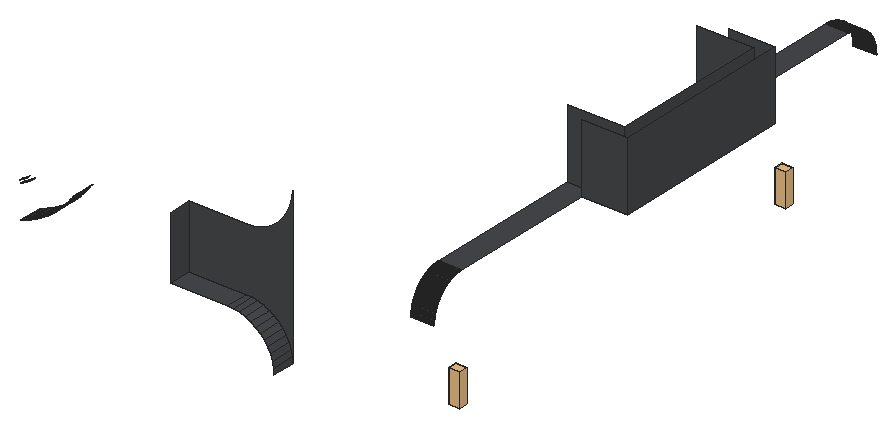
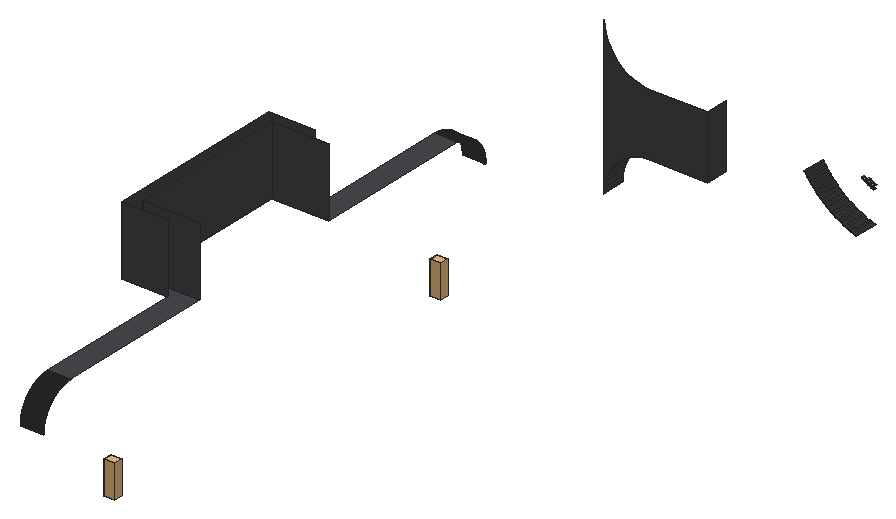
# SketchUp Ruby script. Lengths in inches.
U = 1.inch
M = Sketchup.active_model
def pt(a) = Geom::Point3d.new(a.map { |v| v * U })
def face(e, loops, mat)
  f = e.add_face(loops[0].map { |a| pt(a) })
  loops[1..].each { |l| e.add_face(l.map { |a| pt(a) }).erase! }
  f.material = f.back_material = mat if mat
  f
end
# faces: each face lists its corners as indices into pts; further lists are holes
def faces(e, pts, list, mat = nil) = list.each { |f| face(e, (f[0].is_a?(Array) ? f : [f]).map { |l| l.map { |i| pts[i] } }, mat) }
# xy, xz, yz: faces in a plane at the given z, y or x. An outline is a flat list of corners, or four numbers for a rectangle; further outlines are holes
def ring(l) = l.size == 4 ? [[l[0], l[1]], [l[2], l[1]], [l[2], l[3]], [l[0], l[3]]] : l.each_slice(2).to_a
def flat(e, list, mat, &to3) = list.each { |f| face(e, (f[0].is_a?(Array) ? f : [f]).map { |l| ring(l).map { |u, v| to3.(u, v) } }, mat) }
def xy(e, z, list, mat = nil) = flat(e, list, mat) { |x, y| [x, y, z] }
def xz(e, y, list, mat = nil) = flat(e, list, mat) { |x, z| [x, y, z] }
def yz(e, x, list, mat = nil) = flat(e, list, mat) { |y, z| [x, y, z] }
def lines(e, pts, list) = list.each { |a, b| e.add_line(pt(pts[a]), pt(pts[b])) }
# prism: a flat outline (further loops are holes) pulled along v
def prism(e, loops, v, mat = nil)
  f = face(e, loops, mat); d = Geom::Vector3d.new(v.map { |x| x * U })
  f.pushpull(f.normal.samedirection?(d) ? d.length : -d.length)
end
def box(e, o, s, mat = nil) = prism(e, [[o, [o[0] + s[0], o[1], o[2]], [o[0] + s[0], o[1] + s[1], o[2]], [o[0], o[1] + s[1], o[2]]]], [0, 0, s[2]], mat)
def at(x, y, z, deg = 0) = Geom::Transformation.translation(pt([x, y, z])) * Geom::Transformation.rotation(ORIGIN, Z_AXIS, deg.degrees)
def axes(o, x, y, z) = Geom::Transformation.new([*x, 0, *y, 0, *z, 0, *pt(o).to_a, 1])
def part(name) = M.definitions.add(name)
# library, detail: a bought-in or finely detailed component or shape, given as its bounding box
def library(name, o, s) = part(name).tap { |d| box(d.entities, o, s) }
def detail(e, o, s) = box(e.add_group.entities, o, s)
def put(e, d, t, mat = nil) = e.add_instance(d, t).tap { |i| i.material = mat if mat }
def group(e, t, mat = nil) = e.add_group.tap { |g| g.transformation = t; g.material = mat if mat }.entities
root = M.entities
M.materials.add("1432 AP 8245 TAR ROAD").color = [71, 72, 75]
M.materials.add("Outer Light").color = [251, 217, 152]
c1 = library("WALL LIGHT 69",[4.19,4.05,-8.78],[4.61,5.7,17.13])
xy(root,269.79,[[486,95.37,516,107.37]],"1432 AP 8245 TAR ROAD")
xy(root,281.79,[[573,160.9,585,161.13],[573,161.13,585,161.37],[573,161.37,573,245.37,603,245.37,603,329.37,573,329.37,573,413.37,585,413.37,585,335.37,609,335.37,609,239.37,585,239.37,585,161.37],[573,413.37,585,413.61],[573,413.61,585,413.84]],"1432 AP 8245 TAR ROAD")
xz(root,107.37,[[540,245.79,539.79,248.92,539.18,252,538.17,254.98,536.78,257.79,535.04,260.4,532.97,262.76,530.61,264.83,528,266.58,525.18,267.97,522.21,268.97,519.13,269.59,516,269.79,486,269.79,486,302.79,516,302.79,519.13,303,522.21,303.61,525.18,304.62,528,306.01,530.61,307.75,532.97,309.82,535.04,312.18,536.78,314.79,538.17,317.61,539.18,320.58,539.79,323.66,540,326.79]],"1432 AP 8245 TAR ROAD")
xz(root,143.37,[[573,263.79,585,264.03]],"1432 AP 8245 TAR ROAD")
xz(root,239.37,[[585,281.79,609,317.79]],"1432 AP 8245 TAR ROAD")
xz(root,245.37,[[573,281.79,603,317.79]],"1432 AP 8245 TAR ROAD")
xz(root,329.37,[[573,281.79,603,317.79]],"1432 AP 8245 TAR ROAD")
xz(root,335.37,[[585,281.79,609,317.79]],"1432 AP 8245 TAR ROAD")
xz(root,431.36,[[573,264.26,585,264.5]],"1432 AP 8245 TAR ROAD")
xz(root,431.37,[[573,263.79,585,264.03]],"1432 AP 8245 TAR ROAD")
yz(root,486,[[95.37,269.79,107.37,302.79]],"1432 AP 8245 TAR ROAD")
yz(root,603,[[245.37,281.79,329.37,317.79]],"1432 AP 8245 TAR ROAD")
yz(root,609,[[239.37,281.79,335.37,317.79]],"1432 AP 8245 TAR ROAD")
p = [[540,95.37,245.79],[539.79,95.37,248.92],[539.79,107.37,248.92],[540,107.37,245.79],[539.18,95.37,252],[539.18,107.37,252],
  [538.17,95.37,254.98],[538.17,107.37,254.98],[536.78,95.37,257.79],[536.78,107.37,257.79],[535.04,95.37,260.4],[535.04,107.37,260.4],
  [532.97,95.37,262.76],[532.97,107.37,262.76],[530.61,95.37,264.83],[530.61,107.37,264.83],[573,143.37,264.03],[573,143.375,264.26],
  [585,143.375,264.26],[585,143.37,264.03],[573,431.36,264.26],[573,431.37,264.03],[585,431.37,264.03],[585,431.36,264.26],
  [573,143.38,264.5],[585,143.38,264.5],[573,143.39,264.73],[585,143.39,264.73],[573,431.35,264.73],[573,431.36,264.5],
  [585,431.36,264.5],[585,431.35,264.73],[573,143.41,264.97],[585,143.41,264.97],[573,431.33,264.97],[585,431.33,264.97],
  [528,95.37,266.58],[528,107.37,266.58],[573,143.43,265.2],[585,143.43,265.2],[573,431.3125,265.2],[585,431.3125,265.2],
  [573,143.45,265.4375],[585,143.45,265.4375],[573,431.29,265.4375],[585,431.29,265.4375],[573,143.47,265.67],[585,143.47,265.67],
  [573,431.27,265.67],[585,431.27,265.67],[573,143.49,265.91],[585,143.49,265.91],[573,431.25,265.91],[585,431.25,265.91],
  [573,143.52,266.14],[585,143.52,266.14],[573,431.22,266.14],[585,431.22,266.14],[573,143.56,266.375],[585,143.56,266.375],
  [573,431.18,266.375],[585,431.18,266.375],[573,143.59,266.61],[585,143.59,266.61],[573,431.15,266.61],[585,431.15,266.61],
  [525.18,95.37,267.97],[525.18,107.37,267.97],[573,143.63,266.84],[585,143.63,266.84],[573,431.11,266.84],[585,431.11,266.84],
  [573,143.67,267.07],[585,143.67,267.07],[573,431.07,267.07],[585,431.07,267.07],[573,143.72,267.3],[585,143.72,267.3],
  [573,431.02,267.3],[585,431.02,267.3],[573,143.76,267.53],[585,143.76,267.53],[573,430.98,267.53],[585,430.98,267.53],
  [573,143.8125,267.76],[585,143.8125,267.76],[573,430.93,267.76],[585,430.93,267.76],[573,143.87,267.99],[585,143.87,267.99],
  [573,430.87,267.99],[585,430.87,267.99],[522.21,95.37,268.97],[522.21,107.37,268.97],[573,143.92,268.22],[585,143.92,268.22],
  [573,430.82,268.22],[585,430.82,268.22],[573,143.98,268.45],[585,143.98,268.45],[573,430.76,268.45],[585,430.76,268.45],
  [573,144.05,268.68],[585,144.05,268.68],[573,430.69,268.68],[585,430.69,268.68],[573,144.11,268.9],[585,144.11,268.9],
  [573,430.63,268.9],[585,430.63,268.9],[573,144.18,269.13],[585,144.18,269.13],[573,430.56,269.13],[585,430.56,269.13],
  [519.13,95.37,269.59],[519.13,107.37,269.59],[573,144.25,269.35],[585,144.25,269.35],[573,430.49,269.35],[585,430.49,269.35],
  [573,144.33,269.58],[585,144.33,269.58],[573,430.41,269.58],[585,430.41,269.58],[516,95.37,269.79],[516,107.37,269.79],
  [573,144.4,269.8],[585,144.4,269.8],[573,430.34,269.8],[585,430.34,269.8],[573,144.48,270.02],[585,144.48,270.02],
  [573,430.26,270.02],[585,430.26,270.02],[573,144.57,270.24],[585,144.57,270.24],[573,430.17,270.24],[585,430.17,270.24],
  [573,144.65,270.46],[585,144.65,270.46],[573,430.09,270.46],[585,430.09,270.46],[573,144.74,270.68],[585,144.74,270.68],
  [573,430,270.68],[585,430,270.68],[573,144.83,270.9],[585,144.83,270.9],[573,429.91,270.9],[585,429.91,270.9],
  [573,144.93,271.11],[585,144.93,271.11],[573,429.8125,271.11],[585,429.8125,271.11],[573,145.02,271.33],[585,145.02,271.33],
  [573,429.72,271.33],[585,429.72,271.33],[573,145.125,271.54],[585,145.125,271.54],[573,429.62,271.54],[585,429.62,271.54],
  [573,145.23,271.75],[585,145.23,271.75],[573,429.51,271.75],[585,429.51,271.75],[573,145.33,271.96],[585,145.33,271.96],
  [573,429.41,271.96],[585,429.41,271.96],[573,145.44,272.17],[585,145.44,272.17],[573,429.3,272.17],[585,429.3,272.17],
  [408.125,107.37,272.09],[408.76,107.37,272.29],[408.76,95.37,272.29],[408.125,95.37,272.09],[573,145.55,272.38],[585,145.55,272.38],
  [573,429.1875,272.38],[585,429.1875,272.38],[409.39,107.37,272.5],[409.39,95.37,272.5],[573,145.67,272.59],[585,145.67,272.59],
  [573,429.07,272.59],[585,429.07,272.59],[410.02,107.37,272.72],[410.02,95.37,272.72],[573,145.78,272.79],[585,145.78,272.79],
  [573,428.96,272.79],[585,428.96,272.79],[410.65,107.37,272.94],[410.65,95.37,272.94],[573,145.9,273],[585,145.9,273],
  [573,428.84,273],[585,428.84,273],[411.28,107.37,273.18],[411.28,95.37,273.18],[573,146.02,273.2],[585,146.02,273.2],
  [573,428.72,273.2],[585,428.72,273.2],[411.9,107.37,273.42],[411.9,95.37,273.42],[573,146.15,273.4],[585,146.15,273.4],
  [573,428.59,273.4],[585,428.59,273.4],[412.52,107.37,273.67],[412.52,95.37,273.67],[573,146.27,273.6],[585,146.27,273.6],
  [573,428.47,273.6],[585,428.47,273.6],[573,146.4,273.79],[585,146.4,273.79],[573,428.34,273.79],[585,428.34,273.79],
  [413.13,107.37,273.93],[413.13,95.37,273.93],[573,146.54,273.99],[585,146.54,273.99],[573,428.2,273.99],[585,428.2,273.99],
  [413.74,107.37,274.2],[413.74,95.37,274.2],[573,146.67,274.18],[585,146.67,274.18],[573,428.07,274.18],[585,428.07,274.18],
  [414.35,107.37,274.48],[414.35,95.37,274.48],[573,146.81,274.37],[585,146.81,274.37],[573,427.93,274.37],[585,427.93,274.37],
  [573,146.95,274.5625],[585,146.95,274.5625],[573,427.79,274.5625],[585,427.79,274.5625],[414.96,107.37,274.76],[414.96,95.37,274.76],
  [573,147.09,274.75],[585,147.09,274.75],[573,427.65,274.75],[585,427.65,274.75],[573,147.23,274.9375],[585,147.23,274.9375],
  [573,427.51,274.9375],[585,427.51,274.9375],[415.56,107.37,275.05],[415.56,95.37,275.05],[573,147.38,275.12],[585,147.38,275.12],
  [573,427.36,275.12],[585,427.36,275.12],[416.15,107.37,275.35],[416.15,95.37,275.35],[573,147.53,275.3],[585,147.53,275.3],
  [573,427.21,275.3],[585,427.21,275.3],[573,147.68,275.48],[585,147.68,275.48],[573,427.06,275.48],[585,427.06,275.48],
  [416.75,107.37,275.66],[416.75,95.37,275.66],[573,147.84,275.66],[585,147.84,275.66],[573,426.9,275.66],[585,426.9,275.66],
  [417.34,107.37,275.97],[417.34,95.37,275.97],[573,147.99,275.84],[585,147.99,275.84],[573,426.75,275.84],[585,426.75,275.84],
  [573,148.15,276.01],[585,148.15,276.01],[573,426.59,276.01],[585,426.59,276.01],[417.92,107.37,276.29],[417.92,95.37,276.29],
  [573,148.3125,276.18],[585,148.3125,276.18],[573,426.43,276.18],[585,426.43,276.18],[573,148.48,276.35],[585,148.48,276.35],
  [573,426.26,276.35],[585,426.26,276.35],[418.5,107.37,276.625],[418.5,95.37,276.625],[573,148.64,276.52],[585,148.64,276.52],
  [573,426.1,276.52],[585,426.1,276.52],[573,148.81,276.69],[585,148.81,276.69],[573,425.93,276.69],[585,425.93,276.69],
  [419.08,107.37,276.96],[419.08,95.37,276.96],[573,148.98,276.85],[585,148.98,276.85],[573,425.76,276.85],[585,425.76,276.85],
  [573,149.15,277.01],[585,149.15,277.01],[573,425.59,277.01],[585,425.59,277.01],[419.65,107.37,277.31],[419.65,95.37,277.31],
  [573,149.33,277.17],[585,149.33,277.17],[573,425.41,277.17],[585,425.41,277.17],[573,149.5,277.33],[585,149.5,277.33],
  [573,425.24,277.33],[585,425.24,277.33],[420.21,107.37,277.66],[420.21,95.37,277.66],[573,149.68,277.48],[585,149.68,277.48],
  [573,425.06,277.48],[585,425.06,277.48],[573,149.86,277.63],[585,149.86,277.63],[573,424.88,277.63],[585,424.88,277.63],
  [573,150.04,277.78],[585,150.04,277.78],[573,424.7,277.78],[585,424.7,277.78],[420.78,107.37,278.02],[420.78,95.37,278.02],
  [573,150.23,277.93],[585,150.23,277.93],[573,424.51,277.93],[585,424.51,277.93],[573,150.41,278.07],[585,150.41,278.07],
  [573,424.33,278.07],[585,424.33,278.07],[421.33,107.37,278.39],[421.33,95.37,278.39],[573,150.6,278.21],[585,150.6,278.21],
  [573,424.14,278.21],[585,424.14,278.21],[573,150.79,278.35],[585,150.79,278.35],[573,423.95,278.35],[585,423.95,278.35],
  [421.89,107.37,278.76],[421.89,95.37,278.76],[573,150.98,278.49],[585,150.98,278.49],[573,423.76,278.49],[585,423.76,278.49],
  [573,151.17,278.625],[585,151.17,278.625],[573,423.57,278.625],[585,423.57,278.625],[573,151.37,278.76],[585,151.37,278.76],
  [573,423.37,278.76],[585,423.37,278.76],[422.43,107.37,279.14],[422.43,95.37,279.14],[573,151.57,278.89],[585,151.57,278.89],
  [573,423.17,278.89],[585,423.17,278.89],[573,151.76,279.02],[585,151.76,279.02],[573,422.97,279.02],[585,422.97,279.02],
  [573,151.96,279.14],[585,151.96,279.14],[573,422.77,279.14],[585,422.77,279.14],[422.98,107.37,279.53],[422.98,95.37,279.53],
  [573,152.17,279.26],[585,152.17,279.26],[573,422.57,279.26],[585,422.57,279.26],[573,152.37,279.38],[585,152.37,279.38],
  [573,422.37,279.38],[585,422.37,279.38],[573,152.57,279.5],[585,152.57,279.5],[573,422.17,279.5],[585,422.17,279.5],
  [423.51,107.37,279.93],[423.51,95.37,279.93],[573,152.78,279.61],[585,152.78,279.61],[573,421.96,279.61],[585,421.96,279.61],
  [573,152.99,279.72],[585,152.99,279.72],[573,421.75,279.72],[585,421.75,279.72],[573,153.2,279.83],[585,153.2,279.83],
  [573,421.54,279.83],[585,421.54,279.83],[573,153.41,279.9375],[585,153.41,279.9375],[573,421.33,279.9375],[585,421.33,279.9375],
  [424.05,107.37,280.33],[424.05,95.37,280.33],[573,153.62,280.04],[585,153.62,280.04],[573,421.12,280.04],[585,421.12,280.04],
  [573,153.83,280.14],[585,153.83,280.14],[573,420.91,280.14],[585,420.91,280.14],[573,154.05,280.24],[585,154.05,280.24],
  [573,420.69,280.24],[585,420.69,280.24],[573,154.26,280.33],[585,154.26,280.33],[573,420.48,280.33],[585,420.48,280.33],
  [424.57,107.37,280.74],[424.57,95.37,280.74],[573,154.48,280.42],[585,154.48,280.42],[573,420.26,280.42],[585,420.26,280.42],
  [573,154.7,280.51],[585,154.7,280.51],[573,420.04,280.51],[585,420.04,280.51],[573,154.92,280.6],[585,154.92,280.6],
  [573,419.82,280.6],[585,419.82,280.6],[573,155.14,280.68],[585,155.14,280.68],[573,419.6,280.68],[585,419.6,280.68],
  [425.1,107.37,281.16],[425.1,95.37,281.16],[573,155.36,280.76],[585,155.36,280.76],[573,419.38,280.76],[585,419.38,280.76],
  [573,155.58,280.84],[585,155.58,280.84],[573,155.81,280.91],[585,155.81,280.91],[573,418.93,280.91],[573,419.16,280.84],
  [585,419.16,280.84],[585,418.93,280.91],[573,156.03,280.98],[585,156.03,280.98],[573,418.71,280.98],[585,418.71,280.98],
  [573,156.26,281.05],[585,156.26,281.05],[573,418.48,281.05],[585,418.48,281.05],[573,156.48,281.12],[585,156.48,281.12],
  [573,156.71,281.18],[585,156.71,281.18],[573,418.03,281.18],[573,418.26,281.12],[585,418.26,281.12],[585,418.03,281.18],
  [425.61,107.37,281.58],[425.61,95.37,281.58],[573,156.9375,281.24],[585,156.9375,281.24],[573,157.17,281.29],[585,157.17,281.29],
  [573,417.57,281.29],[573,417.8,281.24],[585,417.8,281.24],[585,417.57,281.29],[573,157.4,281.35],[585,157.4,281.35],
  [573,157.63,281.4],[585,157.63,281.4],[573,417.11,281.4],[573,417.34,281.35],[585,417.34,281.35],[585,417.11,281.4],
  [573,157.86,281.45],[585,157.86,281.45],[573,158.09,281.49],[585,158.09,281.49],[573,416.65,281.49],[573,416.88,281.45],
  [585,416.88,281.45],[585,416.65,281.49],[573,158.32,281.53],[585,158.32,281.53],[573,158.55,281.57],[585,158.55,281.57],
  [573,416.1875,281.57],[573,416.42,281.53],[585,416.42,281.53],[585,416.1875,281.57],[426.12,107.37,282.01],[426.12,95.37,282.01],
  [573,158.79,281.61],[585,158.79,281.61],[573,159.02,281.64],[585,159.02,281.64],[573,159.25,281.67],[585,159.25,281.67],
  [573,415.49,281.67],[573,415.72,281.64],[585,415.72,281.64],[585,415.49,281.67],[573,415.95,281.61],[585,415.95,281.61],
  [573,159.49,281.69],[585,159.49,281.69],[573,159.72,281.72],[585,159.72,281.72],[573,159.96,281.74],[585,159.96,281.74],
  [573,160.19,281.75],[585,160.19,281.75],[573,414.55,281.75],[573,414.78,281.74],[585,414.78,281.74],[585,414.55,281.75],
  [573,415.02,281.72],[585,415.02,281.72],[573,415.25,281.69],[585,415.25,281.69],[573,160.43,281.77],[585,160.43,281.77],
  [573,160.66,281.78],[585,160.66,281.78],[573,160.9,281.79],[585,160.9,281.79],[573,413.84,281.79],[573,414.08,281.78],
  [585,414.08,281.78],[585,413.84,281.79],[573,414.3125,281.77],[585,414.3125,281.77],[426.625,107.37,282.45],[426.625,95.37,282.45],
  [427.125,107.37,282.89],[427.125,95.37,282.89],[427.62,107.37,283.34],[427.62,95.37,283.34],[428.11,107.37,283.8],[428.11,95.37,283.8],
  [428.59,107.37,284.26],[428.59,95.37,284.26],[429.0625,107.37,284.73],[429.0625,95.37,284.73],[429.53,107.37,285.2],[429.53,95.37,285.2],
  [429.99,107.37,285.6875],[429.99,95.37,285.6875],[430.45,107.37,286.17],[430.45,95.37,286.17],[430.9,107.37,286.67],[430.9,95.37,286.67],
  [431.34,107.37,287.17],[431.34,95.37,287.17],[431.78,107.37,287.67],[431.78,95.37,287.67],[432.21,107.37,288.18],[432.21,95.37,288.18],
  [432.63,107.37,288.7],[432.63,95.37,288.7],[433.05,107.37,289.22],[433.05,95.37,289.22],[408.07,95.37,289.2],[408.48,95.37,289.4],
  [408.48,96.87,289.4],[408.07,96.87,289.2],[408.07,96.87,289.2],[408.48,96.87,289.4],[408.48,95.37,289.4],[408.07,95.37,289.2],
  [433.46,107.37,289.75],[433.46,95.37,289.75],[408.89,95.37,289.61],[408.89,96.87,289.61],[408.89,96.87,289.61],[408.89,95.37,289.61],
  [409.3,95.37,289.82],[409.3,96.87,289.82],[409.3,96.87,289.82],[409.3,95.37,289.82],[433.86,107.37,290.28],[433.86,95.37,290.28],
  [409.7,95.37,290.03],[409.7,96.87,290.03],[409.7,96.87,290.03],[409.7,95.37,290.03],[410.1,95.37,290.25],[410.1,96.87,290.25],
  [410.1,96.87,290.25],[410.1,95.37,290.25],[410.5,95.37,290.48],[410.5,96.87,290.48],[410.5,96.87,290.48],[410.5,95.37,290.48],
  [434.26,107.37,290.82],[434.26,95.37,290.82],[410.9,95.37,290.71],[410.9,96.87,290.71],[410.9,96.87,290.71],[410.9,95.37,290.71],
  [408.21,96.87,290.94],[407.82,96.87,290.75],[407.82,95.37,290.75],[408.21,95.37,290.94],[411.29,95.37,290.95],[411.29,96.87,290.95],
  [411.29,96.87,290.95],[411.29,95.37,290.95],[434.65,107.37,291.36],[434.65,95.37,291.36],[408.6,96.87,291.14],[408.6,95.37,291.14],
  [408.6,95.37,291.14],[408.21,95.37,290.94],[408.21,96.87,290.94],[408.6,96.87,291.14],[411.68,95.37,291.19],[411.68,96.87,291.19],
  [411.68,96.87,291.19],[411.68,95.37,291.19],[408.98,96.87,291.35],[408.98,95.37,291.35],[408.98,95.37,291.35],[408.98,96.87,291.35],
  [412.0625,95.37,291.4375],[412.0625,96.87,291.4375],[412.0625,96.87,291.4375],[412.0625,95.37,291.4375],[409.37,96.87,291.5625],[409.37,95.37,291.5625],
  [409.37,95.37,291.5625],[409.37,96.87,291.5625],[412.44,95.37,291.69],[412.44,96.87,291.69],[412.44,96.87,291.69],[412.44,95.37,291.69],
  [435.03,107.37,291.91],[435.03,95.37,291.91],[409.75,96.87,291.78],[409.75,95.37,291.78],[409.75,95.37,291.78],[409.75,96.87,291.78],
  [412.82,95.37,291.95],[412.82,96.87,291.95],[412.82,96.87,291.95],[412.82,95.37,291.95],[410.13,96.87,292],[410.13,95.37,292],
  [410.13,95.37,292],[410.13,96.87,292],[413.2,95.37,292.21],[413.2,96.87,292.21],[413.2,96.87,292.21],[413.2,95.37,292.21],
  [435.4,107.37,292.46],[435.4,95.37,292.46],[410.5,96.87,292.23],[410.5,95.37,292.23],[410.5,95.37,292.23],[410.5,96.87,292.23],
  [410.875,96.87,292.46],[410.875,95.37,292.46],[410.875,95.37,292.46],[410.875,96.87,292.46],[413.57,95.37,292.48],[413.57,96.87,292.48],
  [413.57,96.87,292.48],[413.57,95.37,292.48],[411.25,96.87,292.7],[411.25,95.37,292.7],[411.25,95.37,292.7],[411.25,96.87,292.7],
  [413.94,95.37,292.75],[413.94,96.87,292.75],[413.94,96.87,292.75],[413.94,95.37,292.75],[435.77,107.37,293.02],[435.77,95.37,293.02],
  [411.61,96.87,292.9375],[411.61,95.37,292.9375],[411.61,95.37,292.9375],[411.61,96.87,292.9375],[414.31,95.37,293.02],[414.31,96.87,293.02]]
faces(root,p,[[0,1,2,3],[1,4,5,2],[4,6,7,5],[6,8,9,7],[8,10,11,9],[10,12,13,11],[12,14,15,13],[16,17,18,19],
  [20,21,22,23],[17,24,25,18],[24,26,27,25],[28,29,30,31],[26,32,33,27],[34,28,31,35],[14,36,37,15],[32,38,39,33],
  [40,34,35,41],[38,42,43,39],[44,40,41,45],[42,46,47,43],[48,44,45,49],[46,50,51,47],[52,48,49,53],[50,54,55,51],
  [56,52,53,57],[54,58,59,55],[60,56,57,61],[58,62,63,59],[64,60,61,65],[36,66,67,37],[62,68,69,63],[70,64,65,71],
  [68,72,73,69],[74,70,71,75],[72,76,77,73],[78,74,75,79],[76,80,81,77],[82,78,79,83],[80,84,85,81],[86,82,83,87],
  [84,88,89,85],[90,86,87,91],[66,92,93,67],[88,94,95,89],[96,90,91,97],[94,98,99,95],[100,96,97,101],[98,102,103,99],
  [104,100,101,105],[102,106,107,103],[108,104,105,109],[106,110,111,107],[112,108,109,113],[92,114,115,93],[110,116,117,111],[118,112,113,119],
  [116,120,121,117],[122,118,119,123],[114,124,125,115],[120,126,127,121],[128,122,123,129],[126,130,131,127],[132,128,129,133],[130,134,135,131],
  [136,132,133,137],[134,138,139,135],[140,136,137,141],[138,142,143,139],[144,140,141,145],[142,146,147,143],[148,144,145,149],[146,150,151,147],
  [152,148,149,153],[150,154,155,151],[156,152,153,157],[154,158,159,155],[160,156,157,161],[158,162,163,159],[164,160,161,165],[162,166,167,163],
  [168,164,165,169],[166,170,171,167],[172,168,169,173],[174,175,176,177],[170,178,179,171],[180,172,173,181],[175,182,183,176],[178,184,185,179],
  [186,180,181,187],[182,188,189,183],[184,190,191,185],[192,186,187,193],[188,194,195,189],[190,196,197,191],[198,192,193,199],[194,200,201,195],
  [196,202,203,197],[204,198,199,205],[200,206,207,201],[202,208,209,203],[210,204,205,211],[206,212,213,207],[208,214,215,209],[216,210,211,217],
  [214,218,219,215],[220,216,217,221],[212,222,223,213],[218,224,225,219],[226,220,221,227],[222,228,229,223],[224,230,231,225],[232,226,227,233],
  [228,234,235,229],[230,236,237,231],[238,232,233,239],[236,240,241,237],[242,238,239,243],[234,244,245,235],[240,246,247,241],[248,242,243,249],
  [246,250,251,247],[252,248,249,253],[244,254,255,245],[250,256,257,251],[258,252,253,259],[254,260,261,255],[256,262,263,257],[264,258,259,265],
  [262,266,267,263],[268,264,265,269],[260,270,271,261],[266,272,273,267],[274,268,269,275],[270,276,277,271],[272,278,279,273],[280,274,275,281],
  [278,282,283,279],[284,280,281,285],[276,286,287,277],[282,288,289,283],[290,284,285,291],[288,292,293,289],[294,290,291,295],[286,296,297,287],
  [292,298,299,293],[300,294,295,301],[298,302,303,299],[304,300,301,305],[296,306,307,297],[302,308,309,303],[310,304,305,311],[308,312,313,309],
  [314,310,311,315],[306,316,317,307],[312,318,319,313],[320,314,315,321],[318,322,323,319],[324,320,321,325],[316,326,327,317],[322,328,329,323],
  [330,324,325,331],[328,332,333,329],[334,330,331,335],[332,336,337,333],[338,334,335,339],[326,340,341,327],[336,342,343,337],[344,338,339,345],
  [342,346,347,343],[348,344,345,349],[340,350,351,341],[346,352,353,347],[354,348,349,355],[352,356,357,353],[358,354,355,359],[350,360,361,351],
  [356,362,363,357],[364,358,359,365],[362,366,367,363],[368,364,365,369],[366,370,371,367],[372,368,369,373],[360,374,375,361],[370,376,377,371],
  [378,372,373,379],[376,380,381,377],[382,378,379,383],[380,384,385,381],[386,382,383,387],[374,388,389,375],[384,390,391,385],[392,386,387,393],
  [390,394,395,391],[396,392,393,397],[394,398,399,395],[400,396,397,401],[388,402,403,389],[398,404,405,399],[406,400,401,407],[404,408,409,405],
  [410,406,407,411],[408,412,413,409],[414,410,411,415],[412,416,417,413],[418,414,415,419],[402,420,421,403],[416,422,423,417],[424,418,419,425],
  [422,426,427,423],[428,424,425,429],[426,430,431,427],[432,428,429,433],[430,434,435,431],[436,432,433,437],[420,438,439,421],[434,440,441,435],
  [442,436,437,443],[440,444,445,441],[446,442,443,447],[444,448,449,445],[450,446,447,451],[448,452,453,449],[454,450,451,455],[438,456,457,439],
  [452,458,459,453],[460,454,455,461],[458,462,463,459],[462,464,465,463],[466,467,468,469],[467,460,461,468],[464,470,471,465],[472,466,469,473],
  [470,474,475,471],[476,472,473,477],[474,478,479,475],[478,480,481,479],[482,483,484,485],[483,476,477,484],[456,486,487,457],[480,488,489,481],
  [488,490,491,489],[492,493,494,495],[493,482,485,494],[490,496,497,491],[496,498,499,497],[500,501,502,503],[501,492,495,502],[498,504,505,499],
  [504,506,507,505],[508,509,510,511],[509,500,503,510],[506,512,513,507],[512,514,515,513],[516,517,518,519],[517,508,511,518],[486,520,521,487],
  [514,522,523,515],[522,524,525,523],[524,526,527,525],[528,529,530,531],[529,532,533,530],[532,516,519,533],[526,534,535,527],[534,536,537,535],
  [536,538,539,537],[538,540,541,539],[542,543,544,545],[543,546,547,544],[546,548,549,547],[548,528,531,549],[540,550,551,541],[550,552,553,551],
  [552,554,555,553],[556,557,558,559],[557,560,561,558],[560,542,545,561],[520,562,563,521],[562,564,565,563],[564,566,567,565],[566,568,569,567],
  [568,570,571,569],[570,572,573,571],[572,574,575,573],[574,576,577,575],[576,578,579,577],[578,580,581,579],[580,582,583,581],[582,584,585,583],
  [584,586,587,585],[586,588,589,587],[588,590,591,589],[592,593,594,595],[590,600,601,591],[593,602,603,594],[602,606,607,603],[600,610,611,601],
  [606,612,613,607],[612,616,617,613],[616,620,621,617],[610,624,625,611],[620,626,627,621],[626,634,635,627],[624,638,639,625],[642,643,644,645],
  [634,646,647,635],[652,642,645,653],[646,654,655,647],[660,652,653,661],[654,662,663,655],[638,666,667,639],[670,660,661,671],[662,672,673,663],
  [678,670,671,679],[672,680,681,673],[666,684,685,667],[688,678,679,689],[692,688,689,693],[680,694,695,681],[700,692,693,701],[694,702,703,695],
  [684,706,707,685],[710,700,701,711],[702,712,713,703]],"1432 AP 8245 TAR ROAD")
faces(root,p,[[596,597,598,599],[597,604,605,598],[604,608,609,605],[608,614,615,609],[614,618,619,615],[618,622,623,619],[622,628,629,623],[630,631,632,633],
  [628,636,637,629],[640,630,633,641],[636,648,649,637],[650,640,641,651],[648,656,657,649],[658,650,651,659],[656,664,665,657],[668,658,659,669],
  [664,674,675,665],[676,668,669,677],[674,682,683,675],[686,676,677,687],[690,686,687,691],[682,696,697,683],[698,690,691,699],[696,704,705,697],
  [708,698,699,709]],"Outer Light")
put(root,c1,at(583.25,162.99,221.35,90))
put(root,c1,at(583.25,375.38,221.35,90))
